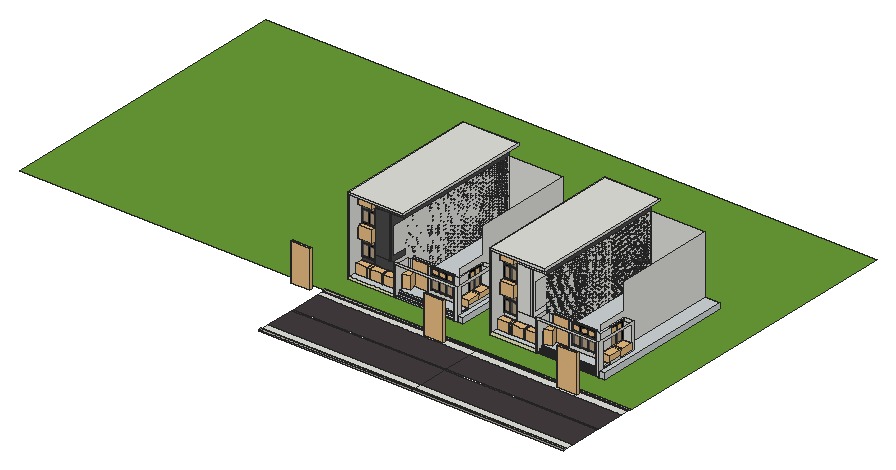
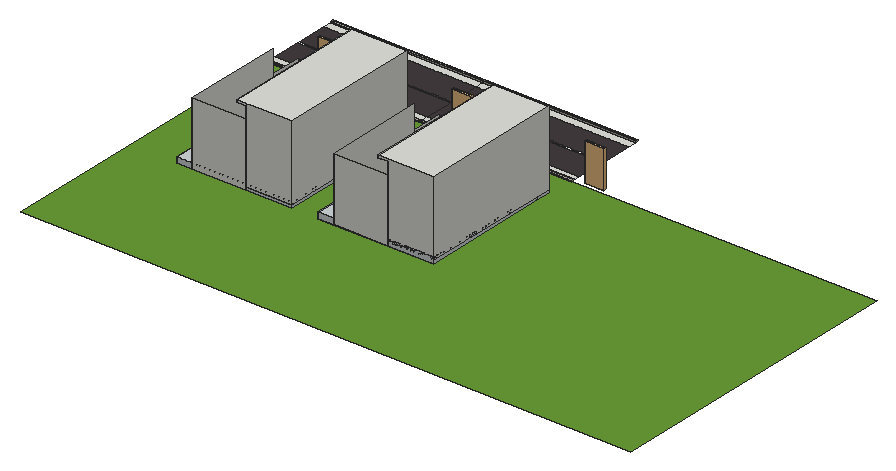
# SketchUp Ruby script. Lengths in inches.
U = 1.inch
M = Sketchup.active_model
def pt(a) = Geom::Point3d.new(a.map { |v| v * U })
def face(e, loops, mat)
  f = e.add_face(loops[0].map { |a| pt(a) })
  loops[1..].each { |l| e.add_face(l.map { |a| pt(a) }).erase! }
  f.material = f.back_material = mat if mat
  f
end
# faces: each face lists its corners as indices into pts; further lists are holes
def faces(e, pts, list, mat = nil) = list.each { |f| face(e, (f[0].is_a?(Array) ? f : [f]).map { |l| l.map { |i| pts[i] } }, mat) }
# xy, xz, yz: faces in a plane at the given z, y or x. An outline is a flat list of corners, or four numbers for a rectangle; further outlines are holes
def ring(l) = l.size == 4 ? [[l[0], l[1]], [l[2], l[1]], [l[2], l[3]], [l[0], l[3]]] : l.each_slice(2).to_a
def flat(e, list, mat, &to3) = list.each { |f| face(e, (f[0].is_a?(Array) ? f : [f]).map { |l| ring(l).map { |u, v| to3.(u, v) } }, mat) }
def xy(e, z, list, mat = nil) = flat(e, list, mat) { |x, y| [x, y, z] }
def xz(e, y, list, mat = nil) = flat(e, list, mat) { |x, z| [x, y, z] }
def yz(e, x, list, mat = nil) = flat(e, list, mat) { |y, z| [x, y, z] }
def lines(e, pts, list) = list.each { |a, b| e.add_line(pt(pts[a]), pt(pts[b])) }
# prism: a flat outline (further loops are holes) pulled along v
def prism(e, loops, v, mat = nil)
  f = face(e, loops, mat); d = Geom::Vector3d.new(v.map { |x| x * U })
  f.pushpull(f.normal.samedirection?(d) ? d.length : -d.length)
end
def box(e, o, s, mat = nil) = prism(e, [[o, [o[0] + s[0], o[1], o[2]], [o[0] + s[0], o[1] + s[1], o[2]], [o[0], o[1] + s[1], o[2]]]], [0, 0, s[2]], mat)
def at(x, y, z, deg = 0) = Geom::Transformation.translation(pt([x, y, z])) * Geom::Transformation.rotation(ORIGIN, Z_AXIS, deg.degrees)
def axes(o, x, y, z) = Geom::Transformation.new([*x, 0, *y, 0, *z, 0, *pt(o).to_a, 1])
def part(name) = M.definitions.add(name)
# library, detail: a bought-in or finely detailed component or shape, given as its bounding box
def library(name, o, s) = part(name).tap { |d| box(d.entities, o, s) }
def detail(e, o, s) = box(e.add_group.entities, o, s)
def put(e, d, t, mat = nil) = e.add_instance(d, t).tap { |i| i.material = mat if mat }
def group(e, t, mat = nil) = e.add_group.tap { |g| g.transformation = t; g.material = mat if mat }.entities
root = M.entities
M.materials.add("1408 AP K082 Hot Ganache-N").color = [74, 72, 72]
M.materials.add("Polycor-Pavers-GEORGIA-MARBLEtm-PEARL-GREY-Tranche-1-4K").color = [207, 214, 215]
M.materials.add("Teddy_Paper").color = [237, 237, 189]
M.materials.add("[Asphalt_New]").color = [67, 60, 62]
M.materials.add("[Color M09]").color = [0, 0, 0]
M.materials.add("[Color_000]").color = [255, 255, 255]
M.materials.add("[Grass Dark Green]").color = [106, 157, 55]
M.materials.add("[Stone_Masonry_Multi]").color = [182, 175, 164]
M.materials.add("[Translucent Glass Gray]").color = [128, 128, 128]
M.materials["[Translucent Glass Gray]"].alpha = 0.5
c1 = library("Street Lighting Pole",[31.3125,-4.22,0],[127.34,10.44,259.08])
c2 = library("Group13",[-203.48,36.63,0],[29.68,67.31,50.64])
c3 = library("Group13\#2",[-203.48,36.63,0],[29.68,67.31,50.64])
c4 = part("Group\#61")
p = [[0,1.89,0.38],[0,1.89,1.61],[0,0.72,0],[0,0,0.99],[0,0.72,1.99]]
lines(c4.entities,p,[[0,1],[2,0],[3,2],[4,3],[1,4]])
c5 = part("Component\#76")
p = [[20.45,2.26,80],[20.78,2.41,80]]
lines(c5.entities,p,[[0,1]])
detail(c5.entities,[0,1.93,2.7],[20.05,3.87,77.3])
put(c5.entities,c4,at(9.77,5.02,80,-180))
put(c5.entities,c4,at(11.91,5.02,80,-180))
put(c5.entities,c4,at(13.54,5.02,80,-180))
put(c5.entities,c4,at(7.29,5.02,80,-180))
put(c5.entities,c4,at(6.18,5.02,80,-180))
put(c5.entities,c4,at(8.69,5.02,80,-180))
put(c5.entities,c4,at(17.42,5.04,80,-180))
put(c5.entities,c4,at(18.86,5.04,80,-180))
put(c5.entities,c4,at(15.09,5.02,80,-180))
put(c5.entities,c4,at(16.66,5.04,80,-180))
put(c5.entities,c4,at(2.54,5.02,80,-180))
put(c5.entities,c4,at(1.38,5.02,80,-180))
put(c5.entities,c4,at(4.1,5.02,80,-180))
c6 = library("Group96\#1",[-28.47,-25.5,0],[56.94,51,19.8125])
c7 = library("Group112\#2",[-28.47,-24.66,0],[56.94,49.32,19.8125])
c8 = library("cay+chuoi",[36.12,19.66,0.52],[32.73,35.6,54.38])
c9 = part("Group\#1")
xy(c9.entities,-18,[[0,0,192,60],[456.375,0,456.375,60,449.99,60,449.99,7.5,442.99,7.5,442.99,1,200.82,1,200.82,60,0,60,0,600,480,600,480,0]])
xy(c9.entities,-12.875,[[7.5,33,184.5,52.5]])
xy(c9.entities,-12,[[200.82,0,442.99,1]])
xy(c9.entities,-10,[[200.82,0,442.99,8.5]],"Polycor-Pavers-GEORGIA-MARBLEtm-PEARL-GREY-Tranche-1-4K")
xy(c9.entities,-5.0625,[[[0,0,192,60],[7.5,33,184.5,52.5]]])
xy(c9.entities,-4,[[200.82,7.5,442.99,8.5]])
xy(c9.entities,-2,[[200.82,7.5,442.99,16]],"Polycor-Pavers-GEORGIA-MARBLEtm-PEARL-GREY-Tranche-1-4K")
xy(c9.entities,4,[[200.82,15,442.99,16]])
xy(c9.entities,6,[[456.375,0,480,0,480,600,0,600,0,60,200.82,60,200.82,15,442.99,15,442.99,7.5,449.99,7.5,449.99,60,456.375,60]],"Polycor-Pavers-GEORGIA-MARBLEtm-PEARL-GREY-Tranche-1-4K")
xz(c9.entities,0,[[456.375,-18,480,6]])
xz(c9.entities,0,[[200.82,-12,442.99,-10]],"Polycor-Pavers-GEORGIA-MARBLEtm-PEARL-GREY-Tranche-1-4K")
xz(c9.entities,0,[[0,-18,192,-5.0625]],"Teddy_Paper")
xz(c9.entities,1,[[200.82,-18,442.99,-12]],"Polycor-Pavers-GEORGIA-MARBLEtm-PEARL-GREY-Tranche-1-4K")
xz(c9.entities,7.5,[[442.99,-18,449.99,6]])
xz(c9.entities,7.5,[[200.82,-4,442.99,-2]],"Polycor-Pavers-GEORGIA-MARBLEtm-PEARL-GREY-Tranche-1-4K")
xz(c9.entities,8.5,[[200.82,-10,442.99,-4]],"Polycor-Pavers-GEORGIA-MARBLEtm-PEARL-GREY-Tranche-1-4K")
xz(c9.entities,15,[[200.82,4,442.99,6]],"Polycor-Pavers-GEORGIA-MARBLEtm-PEARL-GREY-Tranche-1-4K")
xz(c9.entities,16,[[200.82,-2,442.99,4]],"Polycor-Pavers-GEORGIA-MARBLEtm-PEARL-GREY-Tranche-1-4K")
xz(c9.entities,33,[[7.5,-12.875,184.5,-5.0625]])
xz(c9.entities,52.5,[[7.5,-12.875,184.5,-5.0625]])
xz(c9.entities,60,[[0,-18,192,-5.0625],[192,-18,200.82,6],[449.99,-18,456.375,6],[0,-5.0625,192,6]])
xz(c9.entities,600,[[0,-18,480,6]])
yz(c9.entities,0,[[0,-18,60,-5.0625],[60,-18,600,6]])
yz(c9.entities,7.5,[[33,-12.875,52.5,-5.0625]])
yz(c9.entities,184.5,[[33,-12.875,52.5,-5.0625]])
yz(c9.entities,192,[[0,-18,60,-5.0625]])
yz(c9.entities,200.82,[[1,-18,1,-12,0,-12,0,-10,8.5,-10,8.5,-4,7.5,-4,7.5,-2,16,-2,16,4,15,4,15,6,60,6,60,-18]])
yz(c9.entities,442.99,[[1,-18,7.5,-18,7.5,-10,0,-10,0,-12,1,-12],[7.5,-10,8.5,-4],[7.5,-2,7.5,6,15,6,15,4,16,4,16,-2]])
yz(c9.entities,449.99,[[7.5,-18,60,6]])
yz(c9.entities,456.375,[[0,-18,60,6]])
yz(c9.entities,480,[[0,-18,600,6]])
c10 = library("Component",[-22.57,36.53,5.61],[7.19,69.19,99.57])
c11 = part("weg 1")
xy(c11.entities,0,[[119.79,-0.03,149.12,635.01],[405.36,-0.03,441.44,635.01]])
xy(c11.entities,0,[[149.12,-0.03,272.68,635.01],[272.68,-0.03,280.61,79.35],[280.61,-0.03,405.36,635.01],[272.68,158.73,280.61,238.11],[272.68,317.49,280.61,396.87],
  [272.68,476.25,280.61,555.63]],"[Asphalt_New]")
xy(c11.entities,0,[[272.68,79.35,280.61,158.73],[272.68,238.11,280.61,317.49],[272.68,396.87,280.61,476.25],[272.68,555.63,280.61,635.01]],"[Color_000]")
xy(c11.entities,4.33,[[108.17,0,119.79,635.01]],"[Stone_Masonry_Multi]")
xy(c11.entities,5.12,[[441.44,-0.03,453.25,635.01]],"[Stone_Masonry_Multi]")
xz(c11.entities,-0.03,[[441.44,0,453.25,5.12]],"[Stone_Masonry_Multi]")
xz(c11.entities,0,[[108.17,0,119.79,4.33]],"[Stone_Masonry_Multi]")
xz(c11.entities,635.01,[[108.17,0,119.79,4.33],[441.44,0,453.25,5.12]],"[Stone_Masonry_Multi]")
yz(c11.entities,108.17,[[0,0,635.01,4.33]],"[Stone_Masonry_Multi]")
yz(c11.entities,119.79,[[0,0,635.01,4.33]],"[Stone_Masonry_Multi]")
yz(c11.entities,441.44,[[-0.03,0,635.01,5.12]],"[Stone_Masonry_Multi]")
yz(c11.entities,453.25,[[-0.03,0,635.01,5.12]],"[Stone_Masonry_Multi]")
c12 = library("curtain",[-132.09,64.9,20.5],[94.35,4.27,84.68])
c13 = library("Group8",[-183.25,9.15,0],[25.91,56.79,43.93])
xy(root,-4.3125,[[1472.84,449.7,1472.84,1049.7,1697.66,1049.7,1697.66,629.7,1737.22,629.7,1737.22,449.7,1730.83,449.7,1730.83,509.7,1564.35,509.7,1564.35,530.01,1495.16,530.01,1495.16,509.7,1481.66,509.7,1481.66,449.7],[1723.83,449.7,1730.83,457.2],[2062.65,449.7,2062.65,1049.7,2287.48,1049.7,2287.48,629.7,2327.03,629.7,2327.03,449.7,2320.65,449.7,2320.65,509.7,2154.16,509.7,2154.16,530.01,2084.98,530.01,2084.98,509.7,2071.48,509.7,2071.48,449.7],[2313.65,449.7,2320.65,457.2]])
xy(root,-4.3125,[[0.03,345.08,2543.53,1622.71]],"[Grass Dark Green]")
xy(root,19.6875,[[1730.83,468.65,1737.22,509.7],[2320.65,468.65,2327.03,509.7]])
xy(root,22.13,[[1702.45,514.49,1732.43,616.09],[2292.26,514.49,2322.24,616.09]])
xy(root,28.51,[[[1697.66,509.7,1737.22,620.88],[1702.45,514.49,1732.43,616.09]],[[2287.48,509.7,2327.03,620.88],[2292.26,514.49,2322.24,616.09]]])
xy(root,34.1875,[[1577.66,512.7,1610.56,533.7],[1610.56,512.7,1640.77,533.7],[1640.77,512.7,1673.66,533.7],[2167.48,512.7,2200.37,533.7],[2200.37,512.7,2230.58,533.7],
  [2230.58,512.7,2263.48,533.7]])
xy(root,34.1875,[[1577.66,509.7,1673.66,512.7],[2167.48,509.7,2263.48,512.7],[1695.66,559.44,1697.66,590.16],[2285.48,559.44,2287.48,590.16],[1695.66,590.16,1697.66,620.88],
  [2285.48,590.16,2287.48,620.88]],"[Color M09]")
xy(root,34.86,[[1681.23,560.12,1695.66,591.16],[2271.04,560.12,2285.48,591.16],[1681.23,591.16,1695.66,620.2],[2271.04,591.16,2285.48,620.2]])
xy(root,36.86,[[1580.34,509.7,1610.56,511.2],[1613.18,509.7,1640.77,511.2],[1643.6,509.7,1670.99,511.2],[2170.15,509.7,2200.37,511.2],[2202.99,509.7,2230.58,511.2],
  [2233.42,509.7,2260.8,511.2],[1580.34,511.2,1610.56,512.7],[1613.18,511.2,1640.77,512.7],[1643.6,511.2,1670.99,512.7],[2170.15,511.2,2200.37,512.7],
  [2202.99,511.2,2230.58,512.7],[2233.42,511.2,2260.8,512.7],[1695.66,562.12,1696.66,589.16],[1696.66,562.12,1697.66,589.16],[2285.48,562.12,2286.48,589.16],
  [2286.48,562.12,2287.48,589.16],[1695.66,589.16,1697.66,590.16],[2285.48,589.16,2287.48,590.16],[1695.66,590.16,1697.66,591.16],[2285.48,590.16,2287.48,591.16],
  [1695.66,591.16,1696.66,618.2],[1696.66,591.16,1697.66,618.2],[2285.48,591.16,2286.48,618.2],[2286.48,591.16,2287.48,618.2]],"[Color M09]")
xz(root,449.7,[[1472.84,-4.3125,1481.66,-4.3125,1481.66,118.87,1723.83,118.87,1723.83,-4.3125,1737.22,-4.3125,1737.22,127.6875,1472.84,127.6875],[2062.65,-4.3125,2071.48,-4.3125,2071.48,118.87,2313.65,118.87,2313.65,-4.3125,2327.03,-4.3125,2327.03,127.6875,2062.65,127.6875]])
xz(root,457.2,[[1723.83,-4.3125,1730.83,118.87],[2313.65,-4.3125,2320.65,118.87]])
xz(root,468.65,[[1730.83,19.6875,1737.22,118.87],[2320.65,19.6875,2327.03,118.87]])
xz(root,509.7,[[1481.66,-4.3125,1495.16,118.87],[1564.35,-4.3125,1730.83,-4.3125,1730.83,28.51,1697.66,28.51,1697.66,118.87,1673.66,118.87,1673.66,34.1875,1577.66,34.1875,1577.66,118.87,1564.35,118.87],[2071.48,-4.3125,2084.98,118.87],[2154.16,-4.3125,2320.65,-4.3125,2320.65,28.51,2287.48,28.51,2287.48,118.87,2263.48,118.87,2263.48,34.1875,2167.48,34.1875,2167.48,118.87,2154.16,118.87],[1730.83,19.6875,1737.22,28.51],
  [2320.65,19.6875,2327.03,28.51]])
xz(root,509.7,[[[1577.66,34.1875,1673.66,118.87],[1580.34,36.86,1610.56,89.9],[1613.18,36.86,1640.77,89.9],[1643.6,36.86,1670.99,89.9],[1580.34,92.58,1610.56,116.1875],[1613.18,92.58,1640.77,116.1875],[1643.6,92.58,1670.99,116.1875]],[[2167.48,34.1875,2263.48,118.87],[2170.15,36.86,2200.37,89.9],[2202.99,36.86,2230.58,89.9],[2233.42,36.86,2260.8,89.9],[2170.15,92.58,2200.37,116.1875],[2202.99,92.58,2230.58,116.1875],[2233.42,92.58,2260.8,116.1875]]],"[Color M09]")
xz(root,511.2,[[1580.34,36.86,1610.56,89.9],[1613.18,36.86,1640.77,89.9],[1643.6,36.86,1670.99,89.9],[2170.15,36.86,2200.37,89.9],[2202.99,36.86,2230.58,89.9],
  [2233.42,36.86,2260.8,89.9]],"[Translucent Glass Gray]")
xz(root,512.7,[[1610.56,34.1875,1613.18,89.9],[2200.37,34.1875,2202.99,89.9]])
xz(root,512.7,[[1577.66,34.1875,1610.56,36.86],[1613.18,34.1875,1640.77,36.86],[1640.77,34.1875,1643.6,89.9],[1643.6,34.1875,1670.99,36.86],[1670.99,34.1875,1673.66,89.9],
  [2167.48,34.1875,2200.37,36.86],[2202.99,34.1875,2230.58,36.86],[2230.58,34.1875,2233.42,89.9],[2233.42,34.1875,2260.8,36.86],[2260.8,34.1875,2263.48,89.9],
  [1577.66,36.86,1580.34,89.9],[2167.48,36.86,2170.15,89.9]],"[Color M09]")
xz(root,514.49,[[1702.45,22.13,1730.83,28.51],[1730.83,22.13,1732.43,28.51],[2292.26,22.13,2320.65,28.51],[2320.65,22.13,2322.24,28.51]])
xz(root,530.01,[[1495.16,-4.3125,1564.35,118.87],[2084.98,-4.3125,2154.16,118.87]])
xz(root,533.7,[[1577.66,34.1875,1610.56,89.9],[1610.56,34.1875,1640.77,89.9],[1640.77,34.1875,1673.66,89.9],[2167.48,34.1875,2200.37,89.9],[2200.37,34.1875,2230.58,89.9],
  [2230.58,34.1875,2263.48,89.9]])
xz(root,559.44,[[1695.66,34.1875,1697.66,118.87],[2285.48,34.1875,2287.48,118.87]],"[Color M09]")
xz(root,560.12,[[1681.23,34.86,1695.66,89.9],[2271.04,34.86,2285.48,89.9]])
xz(root,561.12,[[1695.66,36.86,1697.66,89.9],[2285.48,36.86,2287.48,89.9]])
xz(root,562.12,[[1695.66,36.86,1696.66,89.9],[1696.66,36.86,1697.66,89.9],[2285.48,36.86,2286.48,89.9],[2286.48,36.86,2287.48,89.9]],"[Color M09]")
xz(root,589.16,[[1695.66,36.86,1696.66,89.9],[1696.66,36.86,1697.66,89.9],[2285.48,36.86,2286.48,89.9],[2286.48,36.86,2287.48,89.9]],"[Color M09]")
xz(root,590.16,[[1695.66,34.1875,1697.66,36.86],[2285.48,34.1875,2287.48,36.86]],"[Color M09]")
xz(root,591.16,[[1695.66,36.86,1696.66,89.9],[1696.66,36.86,1697.66,89.9],[2285.48,36.86,2286.48,89.9],[2286.48,36.86,2287.48,89.9]],"[Color M09]")
xz(root,616.09,[[1702.45,22.13,1732.43,28.51],[2292.26,22.13,2322.24,28.51]])
xz(root,618.2,[[1695.66,36.86,1696.66,89.9],[1696.66,36.86,1697.66,89.9],[2285.48,36.86,2286.48,89.9],[2286.48,36.86,2287.48,89.9]],"[Color M09]")
xz(root,620.2,[[1681.23,34.86,1695.66,89.9],[2271.04,34.86,2285.48,89.9]])
xz(root,620.88,[[1697.66,28.51,1737.22,118.87],[2287.48,28.51,2327.03,118.87]])
xz(root,620.88,[[1695.66,34.1875,1697.66,118.87],[2285.48,34.1875,2287.48,118.87]],"[Color M09]")
xz(root,629.7,[[1697.66,-4.3125,1737.22,127.6875],[2287.48,-4.3125,2327.03,127.6875]])
xz(root,1049.7,[[1472.84,-4.3125,1697.66,259.6875],[2062.65,-4.3125,2287.48,259.6875]])
yz(root,1472.84,[[449.7,-4.3125,449.7,127.6875,509.7,127.6875,509.7,151.6875,449.7,151.6875,449.7,259.6875,1049.7,259.6875,1049.7,-4.3125]])
yz(root,1481.66,[[449.7,-4.3125,509.7,118.87]])
yz(root,1495.16,[[509.7,-4.3125,530.01,118.87]])
yz(root,1564.35,[[509.7,-4.3125,530.01,118.87]])
yz(root,1577.66,[[512.7,34.1875,533.7,89.9]])
yz(root,1577.66,[[509.7,34.1875,512.7,118.87]],"[Color M09]")
yz(root,1580.34,[[509.7,36.86,511.2,89.9],[511.2,36.86,512.7,89.9]],"[Color M09]")
yz(root,1610.56,[[509.7,36.86,511.2,89.9],[511.2,36.86,512.7,89.9]],"[Color M09]")
yz(root,1613.18,[[509.7,36.86,511.2,89.9],[511.2,36.86,512.7,89.9]],"[Color M09]")
yz(root,1640.77,[[509.7,36.86,511.2,89.9],[511.2,36.86,512.7,89.9]],"[Color M09]")
yz(root,1643.6,[[509.7,36.86,511.2,89.9],[511.2,36.86,512.7,89.9]],"[Color M09]")
yz(root,1670.99,[[509.7,36.86,511.2,89.9],[511.2,36.86,512.7,89.9]],"[Color M09]")
yz(root,1673.66,[[512.7,34.1875,533.7,89.9]])
yz(root,1673.66,[[509.7,34.1875,512.7,118.87]],"[Color M09]")
yz(root,1681.23,[[560.12,34.86,591.16,89.9],[591.16,34.86,620.2,89.9]])
yz(root,1695.66,[[562.12,34.86,589.16,36.86]])
yz(root,1695.66,[[[559.44,34.1875,620.88,118.87],[560.12,34.86,620.2,118.1875]],[560.12,34.86,562.12,89.9],[589.16,34.86,590.16,36.86],[590.16,34.86,591.16,36.86],[591.16,34.86,618.2,36.86],
  [618.2,34.86,620.2,89.9],[589.16,36.86,591.16,89.9]],"[Color M09]")
yz(root,1696.66,[[562.12,36.86,589.16,89.9],[591.16,36.86,618.2,89.9]],"[Translucent Glass Gray]")
yz(root,1697.66,[[629.7,-4.3125,1049.7,-4.3125,1049.7,259.6875,629.7,259.6875,629.7,151.6875,509.7,151.6875,509.7,127.6875,629.7,127.6875],[509.7,28.51,620.88,28.51,620.88,34.1875,559.44,34.1875,559.44,118.87,509.7,118.87]])
yz(root,1697.66,[[[559.44,34.1875,590.16,34.1875,590.16,36.86,562.12,36.86,562.12,89.9,589.16,89.9,589.16,36.86,591.16,36.86,591.16,89.9,618.2,89.9,618.2,36.86,590.16,36.86,590.16,34.1875,620.88,34.1875,620.88,118.87,559.44,118.87],[591.16,92.58,618.2,116.1875],[562.12,92.58,589.16,116.1875]]],"[Color M09]")
yz(root,1702.45,[[514.49,22.13,616.09,28.51]])
yz(root,1723.83,[[449.7,-4.3125,457.2,118.87]])
yz(root,1730.83,[[457.2,-4.3125,457.2,118.87,468.65,118.87,468.65,19.6875,509.7,19.6875,509.7,-4.3125]])
yz(root,1732.43,[[514.49,22.13,616.09,28.51]])
yz(root,1737.22,[[[449.7,-4.3125,629.7,127.6875],[468.65,19.6875,468.65,118.87,620.88,118.87,620.88,28.51,509.7,28.51,509.7,19.6875]]])
yz(root,2062.65,[[449.7,-4.3125,449.7,127.6875,509.7,127.6875,509.7,151.6875,449.7,151.6875,449.7,259.6875,1049.7,259.6875,1049.7,-4.3125]])
yz(root,2071.48,[[449.7,-4.3125,509.7,118.87]])
yz(root,2084.98,[[509.7,-4.3125,530.01,118.87]])
yz(root,2154.16,[[509.7,-4.3125,530.01,118.87]])
yz(root,2167.48,[[512.7,34.1875,533.7,89.9]])
yz(root,2167.48,[[509.7,34.1875,512.7,118.87]],"[Color M09]")
yz(root,2170.15,[[509.7,36.86,511.2,89.9],[511.2,36.86,512.7,89.9]],"[Color M09]")
yz(root,2200.37,[[509.7,36.86,511.2,89.9],[511.2,36.86,512.7,89.9]],"[Color M09]")
yz(root,2202.99,[[509.7,36.86,511.2,89.9],[511.2,36.86,512.7,89.9]],"[Color M09]")
yz(root,2230.58,[[509.7,36.86,511.2,89.9],[511.2,36.86,512.7,89.9]],"[Color M09]")
yz(root,2233.42,[[509.7,36.86,511.2,89.9],[511.2,36.86,512.7,89.9]],"[Color M09]")
yz(root,2260.8,[[509.7,36.86,511.2,89.9],[511.2,36.86,512.7,89.9]],"[Color M09]")
yz(root,2263.48,[[512.7,34.1875,533.7,89.9]])
yz(root,2263.48,[[509.7,34.1875,512.7,118.87]],"[Color M09]")
yz(root,2271.04,[[560.12,34.86,591.16,89.9],[591.16,34.86,620.2,89.9]])
yz(root,2285.48,[[562.12,34.86,589.16,36.86]])
yz(root,2285.48,[[[559.44,34.1875,620.88,118.87],[560.12,34.86,620.2,118.1875]],[560.12,34.86,562.12,89.9],[589.16,34.86,590.16,36.86],[590.16,34.86,591.16,36.86],[591.16,34.86,618.2,36.86],
  [618.2,34.86,620.2,89.9],[589.16,36.86,591.16,89.9]],"[Color M09]")
yz(root,2286.48,[[562.12,36.86,589.16,89.9],[591.16,36.86,618.2,89.9]],"[Translucent Glass Gray]")
yz(root,2287.48,[[629.7,-4.3125,1049.7,-4.3125,1049.7,259.6875,629.7,259.6875,629.7,151.6875,509.7,151.6875,509.7,127.6875,629.7,127.6875],[509.7,28.51,620.88,28.51,620.88,34.1875,559.44,34.1875,559.44,118.87,509.7,118.87]])
yz(root,2287.48,[[[559.44,34.1875,590.16,34.1875,590.16,36.86,562.12,36.86,562.12,89.9,589.16,89.9,589.16,36.86,591.16,36.86,591.16,89.9,618.2,89.9,618.2,36.86,590.16,36.86,590.16,34.1875,620.88,34.1875,620.88,118.87,559.44,118.87],[591.16,92.58,618.2,116.1875],[562.12,92.58,589.16,116.1875]]],"[Color M09]")
yz(root,2292.26,[[514.49,22.13,616.09,28.51]])
yz(root,2313.65,[[449.7,-4.3125,457.2,118.87]])
yz(root,2320.65,[[457.2,-4.3125,457.2,118.87,468.65,118.87,468.65,19.6875,509.7,19.6875,509.7,-4.3125]])
yz(root,2322.24,[[514.49,22.13,616.09,28.51]])
yz(root,2327.03,[[[449.7,-4.3125,629.7,127.6875],[468.65,19.6875,468.65,118.87,620.88,118.87,620.88,28.51,509.7,28.51,509.7,19.6875]]])
put(root,c1,axes([1252.03,319.78,-4.3125],[-0.6408,0,0],[0,-1,0],[0,0,0.6]))
put(root,c2,at(1246.55,302.57,-3.77,-90))
put(root,c3,at(1302.3,302.57,-3.77,-90))
g1 = group(root,at(1280.84,509.7,19.6875))
xy(g1,-11.0625,[[0,-60,0,540,192,540,192,0,65.94,0,65.94,2,9,2,9,-60]])
xy(g1,36.75,[[9,2,65.94,5],[35.97,5,65.94,22.6875]])
xy(g1,39.75,[[8.8125,5,35.78,22.6875],[35.78,5,35.97,22.6875]])
xy(g1,39.75,[[12,2,35.97,3.5],[38.97,2,62.94,3.5],[12,3.5,35.97,5],[38.97,3.5,62.94,5]],"[Color M09]")
xy(g1,62.03,[[65.94,0,125.97,2],[125.97,0,131.97,2],[131.97,0,192,2],[65.94,5,66.13,22.6875]])
xy(g1,62.31,[[65.94,0,125.97,2],[131.97,0,192,2]])
xy(g1,85.86,[[8.8125,5,9,22.6875]])
xy(g1,86.04,[[65.94,5,66.13,22.6875]])
xy(g1,86.04,[[12,2,35.97,3.5],[38.97,2,62.94,3.5],[12,3.5,35.97,5],[38.97,3.5,62.94,5]],"[Color M09]")
xy(g1,89.04,[[12,2,35.97,3.5],[38.97,2,62.94,3.5],[12,3.5,35.97,5],[38.97,3.5,62.94,5]],"[Color M09]")
xy(g1,109.875,[[35.97,2,38.97,5]])
xy(g1,109.875,[[12,2,35.97,3.5],[38.97,2,62.94,3.5],[12,3.5,35.97,5],[38.97,3.5,62.94,5]],"[Color M09]")
xy(g1,112.875,[[9,2,65.94,5],[35.97,5,65.94,22.6875]])
xy(g1,113.0625,[[9,5,35.78,22.6875]])
xy(g1,162.1875,[[9,2,65.94,5],[9,5,38.97,22.6875],[38.97,5,65.94,22.6875]])
xy(g1,165.375,[[12,2,35.97,3.5],[38.97,2,62.94,3.5],[12,3.5,35.97,5],[38.97,3.5,62.94,5]],"[Color M09]")
xy(g1,212.9,[[12,2,35.97,3.5],[38.97,2,62.94,3.5],[12,3.5,35.97,5],[38.97,3.5,62.94,5]],"[Color M09]")
xy(g1,215.9,[[12,2,35.97,5],[38.97,2,62.94,3.5],[38.97,3.5,62.94,5]],"[Color M09]")
xy(g1,237,[[12,2,35.97,3.5],[38.97,2,62.94,3.5],[12,3.5,35.97,5],[38.97,3.5,62.94,5]],"[Color M09]")
xy(g1,239.72,[[65.94,0,125.97,2],[131.97,0,192,2]])
xy(g1,240,[[65.94,0,125.97,2],[125.97,0,131.97,2],[131.97,0,192,2],[9,2,65.94,5],[9,5,35.97,22.6875],
  [35.97,5,65.94,22.6875]])
xy(g1,291,[[9,-60,9,2,65.94,2,65.94,0,192,0,192,540,230.1875,540,230.1875,-60]])
xy(g1,300,[[0,-60,230.1875,540]])
xz(g1,-60,[[0,-11.0625,9,-11.0625,9,291,230.1875,291,230.1875,300,0,300]])
xz(g1,0,[[65.94,-11.0625,192,62.03],[65.94,62.31,125.97,239.72],[131.97,62.31,192,239.72],[65.94,240,192,291]],"1408 AP K082 Hot Ganache-N")
xz(g1,2,[[65.94,62.03,125.97,62.31],[125.97,62.03,131.97,240],[131.97,62.03,192,62.31],[65.94,62.31,125.97,239.72],[65.94,239.72,125.97,240],
  [131.97,239.72,192,240]])
xz(g1,2,[[9,-11.0625,65.94,36.75]],"1408 AP K082 Hot Ganache-N")
xz(g1,2,[[[9,36.75,65.94,112.875],[12,39.75,35.97,86.04],[38.97,39.75,62.94,86.04],[12,89.04,12,109.875,62.94,109.875,62.94,89.04,38.97,89.04,38.97,109.875,35.97,109.875,35.97,89.04]],[[9,162.1875,65.94,240],[12,165.375,35.97,212.9],[38.97,165.375,62.94,212.9],[12,215.9,35.97,237],[38.97,215.9,62.94,237]]],"[Color M09]")
xz(g1,3.5,[[12,39.75,35.97,86.04],[38.97,39.75,62.94,86.04],[12,89.04,35.97,109.875],[38.97,89.04,62.94,109.875],[12,165.375,35.97,212.9],
  [38.97,165.375,62.94,212.9],[12,215.4,36.54,237],[38.97,215.9,62.94,237]],"[Translucent Glass Gray]")
xz(g1,5,[[9,36.75,35.97,39.75],[35.97,36.75,38.97,86.04],[38.97,36.75,65.94,39.75],[8.8125,39.75,9,85.86],[9,39.75,12,85.86],
  [35.78,39.75,35.97,86.04],[62.94,39.75,65.94,62.03],[62.94,62.03,65.94,62.31],[65.94,62.03,66.13,62.31],[62.94,62.31,65.94,86.04],
  [65.94,62.31,66.13,86.04],[9,85.86,12,86.04],[12,85.86,35.78,86.04],[9,86.04,35.78,89.04],[35.78,86.04,38.97,86.04,38.97,109.875,35.97,109.875,35.97,89.04,35.78,89.04],
  [38.97,86.04,65.94,89.04],[9,89.04,12,89.23],[12,89.04,35.78,89.23],[35.78,89.04,35.97,109.875],[62.94,89.04,65.94,112.875],
  [9,89.23,12,109.875],[9,109.875,35.78,112.875],[35.78,109.875,35.97,112.875],[35.97,109.875,38.97,112.875],[38.97,109.875,62.94,112.875],
  [9,112.875,35.78,113.0625],[9,162.1875,35.97,165.375],[35.97,162.1875,38.97,212.9],[38.97,162.1875,65.94,165.375],[9,165.375,12,212.9],
  [62.94,165.375,65.94,212.9],[9,212.9,35.97,215.9],[35.97,212.9,38.97,240],[38.97,212.9,65.94,215.9],[9,215.9,12,240],
  [62.94,215.9,65.94,237],[12,237,35.97,240],[38.97,237,65.94,240]])
xz(g1,22.6875,[[35.97,36.75,65.94,36.75,65.94,62.03,66.13,62.03,66.13,86.04,35.97,86.04],[8.8125,39.75,35.78,85.86],[35.78,39.75,35.97,86.04],[9,85.86,35.78,89.23],[35.78,86.04,65.94,86.04,65.94,112.875,35.97,112.875,35.97,89.04,35.78,89.04],
  [35.78,89.04,35.97,109.875],[9,89.23,35.78,113.0625],[9,162.1875,38.97,212.9],[38.97,162.1875,65.94,212.9],[9,212.9,35.97,240],
  [35.97,212.9,65.94,240]])
xz(g1,540,[[0,-11.0625,0,300,230.1875,300,230.1875,291,192,291,192,-11.0625]])
yz(g1,0,[[-60,-11.0625,540,300]])
yz(g1,8.8125,[[5,39.75,22.6875,85.86]])
yz(g1,9,[[-60,-11.0625,2,291],[2,36.75,5,112.875],[5,85.86,22.6875,89.23],[5,89.23,22.6875,113.0625],[2,162.1875,5,240],
  [5,162.1875,22.6875,212.9],[5,212.9,22.6875,240]])
yz(g1,12,[[2,39.75,3.5,86.04],[3.5,39.75,5,86.04],[2,89.04,3.5,109.875],[3.5,89.04,5,109.875],[2,165.375,3.5,212.9],
  [3.5,165.375,5,212.9],[2,215.9,3.5,237],[3.5,215.9,5,237]],"[Color M09]")
yz(g1,35.97,[[5,36.75,22.6875,39.75]])
yz(g1,35.97,[[2,39.75,3.5,86.04],[3.5,39.75,5,86.04],[2,89.04,3.5,109.875],[3.5,89.04,5,109.875],[2,165.375,3.5,212.9],
  [3.5,165.375,5,212.9],[2,215.9,5,237]],"[Color M09]")
yz(g1,38.97,[[2,39.75,3.5,86.04],[3.5,39.75,5,86.04],[2,89.04,3.5,109.875],[3.5,89.04,5,109.875],[2,165.375,3.5,212.9],
  [3.5,165.375,5,212.9],[2,215.9,3.5,237],[3.5,215.9,5,237]],"[Color M09]")
yz(g1,62.94,[[2,39.75,3.5,62.03],[3.5,39.75,5,62.03],[2,62.03,3.5,62.31],[3.5,62.03,5,62.31]])
yz(g1,62.94,[[2,62.31,3.5,86.04],[3.5,62.31,5,86.04],[2,89.04,3.5,109.875],[3.5,89.04,5,109.875],[2,165.375,3.5,212.9],
  [3.5,165.375,5,212.9],[2,215.9,3.5,237],[3.5,215.9,5,237]],"[Color M09]")
yz(g1,65.94,[[0,-11.0625,2,62.03],[2,36.75,5,62.03],[5,36.75,22.6875,62.03],[2,62.03,5,62.31],[0,62.31,2,239.72],
  [2,62.31,5,112.875],[5,86.04,22.6875,112.875],[2,162.1875,5,239.72],[5,162.1875,22.6875,212.9],[5,212.9,22.6875,240],
  [2,239.72,5,240],[0,240,2,291]])
yz(g1,66.13,[[5,62.03,22.6875,62.31],[5,62.31,22.6875,86.04]])
yz(g1,125.97,[[0,62.31,2,239.72]])
yz(g1,131.97,[[0,62.31,2,239.72]])
yz(g1,192,[[0,-11.0625,540,-11.0625,540,291,0,291,0,240,2,240,2,239.72,0,239.72,0,62.31,2,62.31,2,62.03,0,62.03]],"1408 AP K082 Hot Ganache-N")
yz(g1,230.1875,[[-60,291,540,300]])
put(g1,c5,axes([61.93,4.77,37.34],[-2.59641,0,0],[0,0.684,0],[0,0,0.92358]))
put(g1,c5,axes([61.93,4.77,163.7],[-2.59641,0,0],[0,0.684,0],[0,0,0.92358]))
put(g1,c6,axes([37.47,2,265.5],[1,0,0],[0,0,1],[0,-1,0]))
put(g1,c7,axes([37.47,2,137.53],[1,0,0],[0,0,1],[0,-1,0]))
put(root,c3,at(1364.86,302.57,-3.77,-90))
put(root,c8,at(1452.6,449.07,19.875,15))
put(root,c9,at(1280.84,449.7,13.6875),"Polycor-Pavers-GEORGIA-MARBLEtm-PEARL-GREY-Tranche-1-4K")
put(root,c10,at(1458.63,498.54,13.6875,-90))
put(root,c11,at(1270.11,453.25,-4.3125,-90))
put(root,c12,at(1709.75,449.7,13.6875))
put(root,c12,axes([1760.52,641.46,13.01],[0,0.61,0],[-1,0,0],[0,0,1]))
put(root,c13,axes([1953.6,497.25,22.13],[1.38,0,0],[0,1.17,0],[0,0,0.61]))
put(root,c13,axes([1958.85,554.02,22.13],[1.40866,0,0],[0,1,0],[0,0,0.61]))
put(root,c1,axes([1807.21,319.78,-4.3125],[-0.6408,0,0],[0,-1,0],[0,0,0.6]))
put(root,c2,at(1836.36,302.57,-3.77,-90))
put(root,c3,at(1892.11,302.57,-3.77,-90))
g2 = group(root,at(1870.65,509.7,19.6875))
xy(g2,-11.0625,[[0,-60,0,540,192,540,192,0,65.94,0,65.94,2,9,2,9,-60]])
xy(g2,36.75,[[9,2,65.94,5],[35.97,5,65.94,22.6875]])
xy(g2,39.75,[[8.8125,5,35.78,22.6875],[35.78,5,35.97,22.6875]])
xy(g2,39.75,[[12,2,35.97,3.5],[38.97,2,62.94,3.5],[12,3.5,35.97,5],[38.97,3.5,62.94,5]],"[Color M09]")
xy(g2,62.03,[[65.94,0,125.97,2],[125.97,0,131.97,2],[131.97,0,192,2],[65.94,5,66.13,22.6875]])
xy(g2,62.31,[[65.94,0,125.97,2],[131.97,0,192,2]])
xy(g2,85.86,[[8.8125,5,9,22.6875]])
xy(g2,86.04,[[65.94,5,66.13,22.6875]])
xy(g2,86.04,[[12,2,35.97,3.5],[38.97,2,62.94,3.5],[12,3.5,35.97,5],[38.97,3.5,62.94,5]],"[Color M09]")
xy(g2,89.04,[[12,2,35.97,3.5],[38.97,2,62.94,3.5],[12,3.5,35.97,5],[38.97,3.5,62.94,5]],"[Color M09]")
xy(g2,109.875,[[35.97,2,38.97,5]])
xy(g2,109.875,[[12,2,35.97,3.5],[38.97,2,62.94,3.5],[12,3.5,35.97,5],[38.97,3.5,62.94,5]],"[Color M09]")
xy(g2,112.875,[[9,2,65.94,5],[35.97,5,65.94,22.6875]])
xy(g2,113.0625,[[9,5,35.78,22.6875]])
xy(g2,162.1875,[[9,2,65.94,5],[9,5,38.97,22.6875],[38.97,5,65.94,22.6875]])
xy(g2,165.375,[[12,2,35.97,3.5],[38.97,2,62.94,3.5],[12,3.5,35.97,5],[38.97,3.5,62.94,5]],"[Color M09]")
xy(g2,212.9,[[12,2,35.97,3.5],[38.97,2,62.94,3.5],[12,3.5,35.97,5],[38.97,3.5,62.94,5]],"[Color M09]")
xy(g2,215.9,[[12,2,35.97,5],[38.97,2,62.94,3.5],[38.97,3.5,62.94,5]],"[Color M09]")
xy(g2,237,[[12,2,35.97,3.5],[38.97,2,62.94,3.5],[12,3.5,35.97,5],[38.97,3.5,62.94,5]],"[Color M09]")
xy(g2,239.72,[[65.94,0,125.97,2],[131.97,0,192,2]])
xy(g2,240,[[65.94,0,125.97,2],[125.97,0,131.97,2],[131.97,0,192,2],[9,2,65.94,5],[9,5,35.97,22.6875],
  [35.97,5,65.94,22.6875]])
xy(g2,291,[[9,-60,9,2,65.94,2,65.94,0,192,0,192,540,230.1875,540,230.1875,-60]])
xy(g2,300,[[0,-60,230.1875,540]])
xz(g2,-60,[[0,-11.0625,9,-11.0625,9,291,230.1875,291,230.1875,300,0,300]])
xz(g2,0,[[65.94,-11.0625,192,62.03],[65.94,62.31,125.97,239.72],[131.97,62.31,192,239.72],[65.94,240,192,291]])
xz(g2,2,[[9,-11.0625,65.94,36.75],[65.94,62.03,125.97,62.31],[125.97,62.03,131.97,240],[131.97,62.03,192,62.31],[65.94,62.31,125.97,239.72],
  [65.94,239.72,125.97,240],[131.97,239.72,192,240]])
xz(g2,2,[[[9,36.75,65.94,112.875],[12,39.75,35.97,86.04],[38.97,39.75,62.94,86.04],[12,89.04,12,109.875,62.94,109.875,62.94,89.04,38.97,89.04,38.97,109.875,35.97,109.875,35.97,89.04]],[[9,162.1875,65.94,240],[12,165.375,35.97,212.9],[38.97,165.375,62.94,212.9],[12,215.9,35.97,237],[38.97,215.9,62.94,237]]],"[Color M09]")
xz(g2,3.5,[[12,39.75,35.97,86.04],[38.97,39.75,62.94,86.04],[12,89.04,35.97,109.875],[38.97,89.04,62.94,109.875],[12,165.375,35.97,212.9],
  [38.97,165.375,62.94,212.9],[12,215.4,36.54,237],[38.97,215.9,62.94,237]],"[Translucent Glass Gray]")
xz(g2,5,[[9,36.75,35.97,39.75],[35.97,36.75,38.97,86.04],[38.97,36.75,65.94,39.75],[8.8125,39.75,9,85.86],[9,39.75,12,85.86],
  [35.78,39.75,35.97,86.04],[62.94,39.75,65.94,62.03],[62.94,62.03,65.94,62.31],[65.94,62.03,66.13,62.31],[62.94,62.31,65.94,86.04],
  [65.94,62.31,66.13,86.04],[9,85.86,12,86.04],[12,85.86,35.78,86.04],[9,86.04,35.78,89.04],[35.78,86.04,38.97,86.04,38.97,109.875,35.97,109.875,35.97,89.04,35.78,89.04],
  [38.97,86.04,65.94,89.04],[9,89.04,12,89.23],[12,89.04,35.78,89.23],[35.78,89.04,35.97,109.875],[62.94,89.04,65.94,112.875],
  [9,89.23,12,109.875],[9,109.875,35.78,112.875],[35.78,109.875,35.97,112.875],[35.97,109.875,38.97,112.875],[38.97,109.875,62.94,112.875],
  [9,112.875,35.78,113.0625],[9,162.1875,35.97,165.375],[35.97,162.1875,38.97,212.9],[38.97,162.1875,65.94,165.375],[9,165.375,12,212.9],
  [62.94,165.375,65.94,212.9],[9,212.9,35.97,215.9],[35.97,212.9,38.97,240],[38.97,212.9,65.94,215.9],[9,215.9,12,240],
  [62.94,215.9,65.94,237],[12,237,35.97,240],[38.97,237,65.94,240]])
xz(g2,22.6875,[[35.97,36.75,65.94,36.75,65.94,62.03,66.13,62.03,66.13,86.04,35.97,86.04],[8.8125,39.75,35.78,85.86],[35.78,39.75,35.97,86.04],[9,85.86,35.78,89.23],[35.78,86.04,65.94,86.04,65.94,112.875,35.97,112.875,35.97,89.04,35.78,89.04],
  [35.78,89.04,35.97,109.875],[9,89.23,35.78,113.0625],[9,162.1875,38.97,212.9],[38.97,162.1875,65.94,212.9],[9,212.9,35.97,240],
  [35.97,212.9,65.94,240]])
xz(g2,540,[[0,-11.0625,0,300,230.1875,300,230.1875,291,192,291,192,-11.0625]])
yz(g2,0,[[-60,-11.0625,540,300]])
yz(g2,8.8125,[[5,39.75,22.6875,85.86]])
yz(g2,9,[[-60,-11.0625,2,291],[2,36.75,5,112.875],[5,85.86,22.6875,89.23],[5,89.23,22.6875,113.0625],[2,162.1875,5,240],
  [5,162.1875,22.6875,212.9],[5,212.9,22.6875,240]])
yz(g2,12,[[2,39.75,3.5,86.04],[3.5,39.75,5,86.04],[2,89.04,3.5,109.875],[3.5,89.04,5,109.875],[2,165.375,3.5,212.9],
  [3.5,165.375,5,212.9],[2,215.9,3.5,237],[3.5,215.9,5,237]],"[Color M09]")
yz(g2,35.97,[[5,36.75,22.6875,39.75]])
yz(g2,35.97,[[2,39.75,3.5,86.04],[3.5,39.75,5,86.04],[2,89.04,3.5,109.875],[3.5,89.04,5,109.875],[2,165.375,3.5,212.9],
  [3.5,165.375,5,212.9],[2,215.9,5,237]],"[Color M09]")
yz(g2,38.97,[[2,39.75,3.5,86.04],[3.5,39.75,5,86.04],[2,89.04,3.5,109.875],[3.5,89.04,5,109.875],[2,165.375,3.5,212.9],
  [3.5,165.375,5,212.9],[2,215.9,3.5,237],[3.5,215.9,5,237]],"[Color M09]")
yz(g2,62.94,[[2,39.75,3.5,62.03],[3.5,39.75,5,62.03],[2,62.03,3.5,62.31],[3.5,62.03,5,62.31]])
yz(g2,62.94,[[2,62.31,3.5,86.04],[3.5,62.31,5,86.04],[2,89.04,3.5,109.875],[3.5,89.04,5,109.875],[2,165.375,3.5,212.9],
  [3.5,165.375,5,212.9],[2,215.9,3.5,237],[3.5,215.9,5,237]],"[Color M09]")
yz(g2,65.94,[[0,-11.0625,2,62.03],[2,36.75,5,62.03],[5,36.75,22.6875,62.03],[2,62.03,5,62.31],[0,62.31,2,239.72],
  [2,62.31,5,112.875],[5,86.04,22.6875,112.875],[2,162.1875,5,239.72],[5,162.1875,22.6875,212.9],[5,212.9,22.6875,240],
  [2,239.72,5,240],[0,240,2,291]])
yz(g2,66.13,[[5,62.03,22.6875,62.31],[5,62.31,22.6875,86.04]])
yz(g2,125.97,[[0,62.31,2,239.72]])
yz(g2,131.97,[[0,62.31,2,239.72]])
yz(g2,192,[[0,-11.0625,540,-11.0625,540,291,0,291,0,240,2,240,2,239.72,0,239.72,0,62.31,2,62.31,2,62.03,0,62.03]],"1408 AP K082 Hot Ganache-N")
yz(g2,230.1875,[[-60,291,540,300]])
put(g2,c5,axes([61.93,4.77,37.34],[-2.59641,0,0],[0,0.684,0],[0,0,0.92358]))
put(g2,c5,axes([61.93,4.77,163.7],[-2.59641,0,0],[0,0.684,0],[0,0,0.92358]))
put(g2,c6,axes([37.47,2,265.5],[1,0,0],[0,0,1],[0,-1,0]))
put(g2,c7,axes([37.47,2,137.53],[1,0,0],[0,0,1],[0,-1,0]))
put(root,c3,at(1954.68,302.57,-3.77,-90))
put(root,c8,at(2042.41,449.07,19.875,15))
put(root,c9,at(1870.65,449.7,13.6875),"Polycor-Pavers-GEORGIA-MARBLEtm-PEARL-GREY-Tranche-1-4K")
put(root,c10,at(2048.44,498.54,13.6875,-90))
put(root,c12,at(2299.57,449.7,13.6875))
put(root,c11,at(1905.15,453.25,-4.3125,-90))
put(root,c12,axes([2350.33,641.46,13.01],[0,0.61,0],[-1,0,0],[0,0,1]))
put(root,c1,axes([2362.4,319.78,-4.3125],[-0.6408,0,0],[0,-1,0],[0,0,0.6]))
put(root,c13,axes([2543.42,497.25,22.13],[1.38,0,0],[0,1.17,0],[0,0,0.61]))
put(root,c13,axes([2548.67,554.02,22.13],[1.40866,0,0],[0,1,0],[0,0,0.61]))
